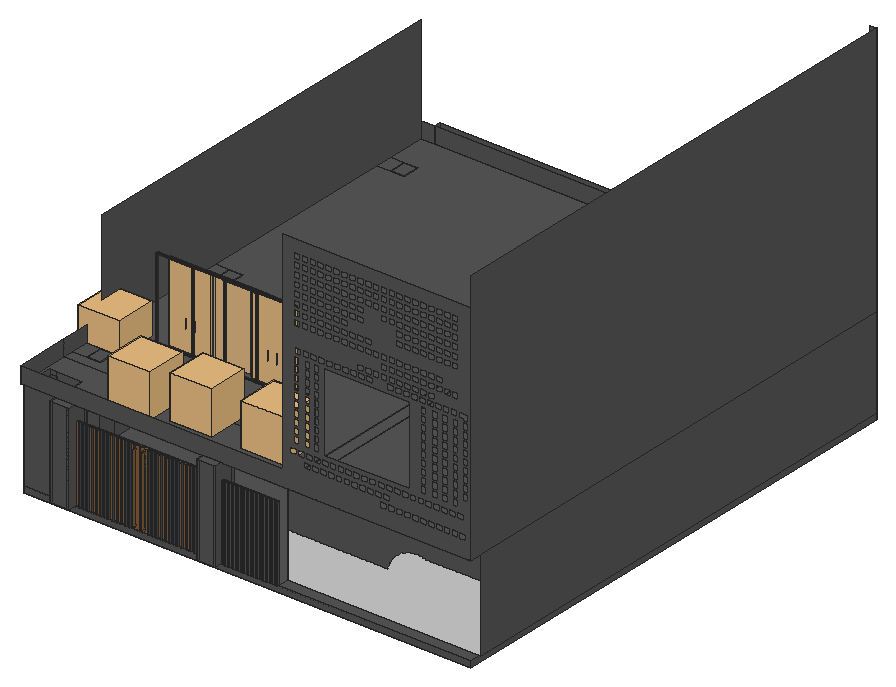
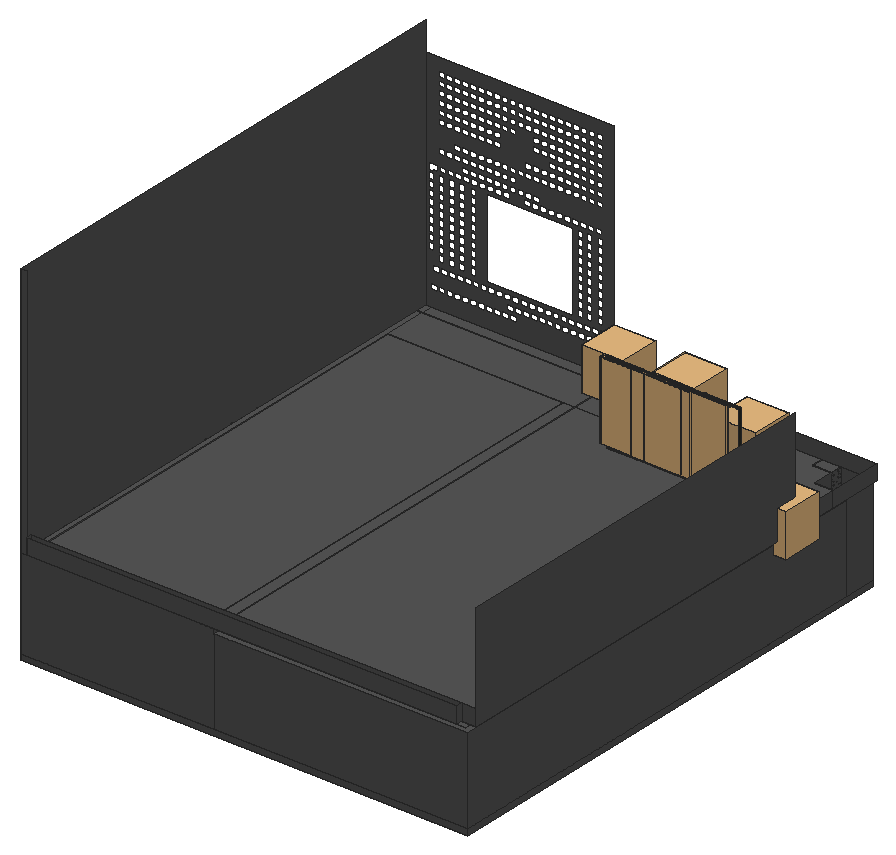
# SketchUp Ruby script. Lengths in inches.
U = 1.inch
M = Sketchup.active_model
def pt(a) = Geom::Point3d.new(a.map { |v| v * U })
def face(e, loops, mat)
  f = e.add_face(loops[0].map { |a| pt(a) })
  loops[1..].each { |l| e.add_face(l.map { |a| pt(a) }).erase! }
  f.material = f.back_material = mat if mat
  f
end
# faces: each face lists its corners as indices into pts; further lists are holes
def faces(e, pts, list, mat = nil) = list.each { |f| face(e, (f[0].is_a?(Array) ? f : [f]).map { |l| l.map { |i| pts[i] } }, mat) }
# xy, xz, yz: faces in a plane at the given z, y or x. An outline is a flat list of corners, or four numbers for a rectangle; further outlines are holes
def ring(l) = l.size == 4 ? [[l[0], l[1]], [l[2], l[1]], [l[2], l[3]], [l[0], l[3]]] : l.each_slice(2).to_a
def flat(e, list, mat, &to3) = list.each { |f| face(e, (f[0].is_a?(Array) ? f : [f]).map { |l| ring(l).map { |u, v| to3.(u, v) } }, mat) }
def xy(e, z, list, mat = nil) = flat(e, list, mat) { |x, y| [x, y, z] }
def xz(e, y, list, mat = nil) = flat(e, list, mat) { |x, z| [x, y, z] }
def yz(e, x, list, mat = nil) = flat(e, list, mat) { |y, z| [x, y, z] }
def lines(e, pts, list) = list.each { |a, b| e.add_line(pt(pts[a]), pt(pts[b])) }
# prism: a flat outline (further loops are holes) pulled along v
def prism(e, loops, v, mat = nil)
  f = face(e, loops, mat); d = Geom::Vector3d.new(v.map { |x| x * U })
  f.pushpull(f.normal.samedirection?(d) ? d.length : -d.length)
end
def box(e, o, s, mat = nil) = prism(e, [[o, [o[0] + s[0], o[1], o[2]], [o[0] + s[0], o[1] + s[1], o[2]], [o[0], o[1] + s[1], o[2]]]], [0, 0, s[2]], mat)
def at(x, y, z, deg = 0) = Geom::Transformation.translation(pt([x, y, z])) * Geom::Transformation.rotation(ORIGIN, Z_AXIS, deg.degrees)
def axes(o, x, y, z) = Geom::Transformation.new([*x, 0, *y, 0, *z, 0, *pt(o).to_a, 1])
def part(name) = M.definitions.add(name)
# library, detail: a bought-in or finely detailed component or shape, given as its bounding box
def library(name, o, s) = part(name).tap { |d| box(d.entities, o, s) }
def detail(e, o, s) = box(e.add_group.entities, o, s)
def put(e, d, t, mat = nil) = e.add_instance(d, t).tap { |i| i.material = mat if mat }
def group(e, t, mat = nil) = e.add_group.tap { |g| g.transformation = t; g.material = mat if mat }.entities
root = M.entities
M.materials.add("48,62,1").color = [75, 79, 82]
M.materials.add("Glazing").color = [128, 128, 128]
M.materials["Glazing"].alpha = 0.05
M.materials.add("Powdercoating").color = [41, 44, 40]
M.materials.add("[Color M06]").color = [86, 86, 86]
M.materials.add("[Polished Concrete Old]").color = [229, 229, 229]
M.materials.add("hpl-fundermax-sheets-500x500").color = [131, 93, 58]
c1 = part("FLUTED+WOOD")
g1 = group(c1.entities,at(0,-21.52,1.9375))
prism(g1,[[[0,45.2,-1.9375],[0.5,45.2,-1.9375],[1,45.2,-1.9375],[1,21.53,-1.9375],[0.5,21.52,-1.9375],[0,21.52,-1.9375],[0,22.6,-1.9375],[0.5,22.6,-1.9375],[0.5,23.14,-1.9375],[0,23.14,-1.9375],[0,24.22,-1.9375],[0.5,24.22,-1.9375],[0.5,24.75,-1.9375],[0,24.75,-1.9375],[0,25.83,-1.9375],[0.5,25.83,-1.9375],[0.5,26.37,-1.9375],[0,26.37,-1.9375],[0,27.44,-1.9375],[0.5,27.44,-1.9375],[0.5,27.98,-1.9375],[0,27.98,-1.9375],[0,29.06,-1.9375],[0.5,29.06,-1.9375],[0.5,29.6,-1.9375],[0,29.6,-1.9375],[0,30.67,-1.9375],[0.5,30.67,-1.9375],[0.5,31.21,-1.9375],[0,31.21,-1.9375],[0,32.29,-1.9375],[0.5,32.29,-1.9375],[0.5,32.83,-1.9375],[0,32.83,-1.9375],[0,33.9,-1.9375],[0.5,33.9,-1.9375],[0.5,34.44,-1.9375],[0,34.44,-1.9375],[0,35.52,-1.9375],[0.5,35.52,-1.9375],[0.5,36.05,-1.9375],[0,36.05,-1.9375],[0,37.13,-1.9375],[0.5,37.13,-1.9375],[0.5,37.67,-1.9375],[0,37.67,-1.9375],[0,38.75,-1.9375],[0.5,38.74,-1.9375],[0.5,39.28,-1.9375],[0,39.28,-1.9375],[0,40.36,-1.9375],[0.5,40.36,-1.9375],[0.5,40.9,-1.9375],[0,40.9,-1.9375],[0,41.97,-1.9375],[0.5,41.97,-1.9375],[0.5,42.51,-1.9375],[0,42.51,-1.9375],[0,43.59,-1.9375],[0.5,43.59,-1.9375],[0.5,44.125,-1.9375],[0,44.125,-1.9375]]],[0,0,46.125])
c2 = part("Group\#60")
prism(c2.entities,[[[-0.75,0,69],[-0.75,0,68],[-0.75,-1.375,68],[-0.75,-1.375,4],[-0.75,0,4],[-0.75,0,3],[-0.75,-2.75,3],[-0.75,-2.75,69]]],[1.5,0,0])
c3 = part("Group\#59")
box(c3.entities,[0,-0.75,0],[0.75,0.75,72])
c4 = part("Gate")
g2 = group(c4.entities,at(0,0,0))
g3 = group(g2,at(12,3,0))
prism(g3,[[[1.5,-3,0],[3,-3,0],[3,12,0],[-12,12,0],[-12,-3,0],[-10.5,-3,0]]],[0,0,72])
prism(g3,[[[118.5,-3,0],[120,-3,0],[120,12,0],[105,12,0],[105,-3,0],[106.5,-3,0]]],[0,0,72])
g4 = group(g2,at(121,6.75,0),"hpl-fundermax-sheets-500x500")
xy(g4,0,[[-106.75,0,-55.38,2],[-54.93,0,-4,2]])
xy(g4,60,[[-106.75,0,-55.38,2],[-54.93,0,-4,2]])
xz(g4,0,[[-106.75,0,-59.6,60],[-58.9375,0,-55.38,60],[-54.93,0,-51.375,60],[-50.71,0,-48.04,60],[-47.37,0,-4,60]])
xz(g4,0,[[-59.6,0,-58.9375,60],[-51.375,0,-50.71,60]],"48,62,1")
xz(g4,2,[[-106.75,0,-55.38,60],[-54.93,0,-4,60]])
yz(g4,-106.75,[[0,0,2,60]])
yz(g4,-55.38,[[0,0,2,60]])
yz(g4,-54.93,[[0,0,2,60]])
yz(g4,-4,[[0,0,2,60]])
put(g4,c2,axes([-51.6,0,0],[-0.88961,0,0],[0,1,0],[0,0,0.83333]))
put(g4,c2,axes([-58.71,0,0],[-0.88961,0,0],[0,1,0],[0,0,0.83333]))
put(g4,c3,axes([-47.37,0,0],[-0.88961,0,0],[0,1,0],[0,0,0.83333]),"48,62,1")
put(g4,c3,axes([-44.04,0,0],[-0.88961,0,0],[0,1,0],[0,0,0.83333]),"48,62,1")
put(g4,c3,axes([-40.7,0,0],[-0.88961,0,0],[0,1,0],[0,0,0.83333]),"48,62,1")
put(g4,c3,axes([-37.36,0,0],[-0.88961,0,0],[0,1,0],[0,0,0.83333]),"48,62,1")
put(g4,c3,axes([-34.03,0,0],[-0.88961,0,0],[0,1,0],[0,0,0.83333]),"48,62,1")
put(g4,c3,axes([-30.69,0,0],[-0.88961,0,0],[0,1,0],[0,0,0.83333]),"48,62,1")
put(g4,c3,axes([-27.36,0,0],[-0.88961,0,0],[0,1,0],[0,0,0.83333]),"48,62,1")
put(g4,c3,axes([-24.02,0,0],[-0.88961,0,0],[0,1,0],[0,0,0.83333]),"48,62,1")
put(g4,c3,axes([-20.68,0,0],[-0.88961,0,0],[0,1,0],[0,0,0.83333]),"48,62,1")
put(g4,c3,axes([-17.35,0,0],[-0.88961,0,0],[0,1,0],[0,0,0.83333]),"48,62,1")
put(g4,c3,axes([-14.01,0,0],[-0.88961,0,0],[0,1,0],[0,0,0.83333]),"48,62,1")
put(g4,c3,axes([-10.68,0,0],[-0.88961,0,0],[0,1,0],[0,0,0.83333]),"48,62,1")
put(g4,c3,axes([-7.34,0,0],[-0.88961,0,0],[0,1,0],[0,0,0.83333]),"48,62,1")
put(g4,c3,axes([-4,0,0],[-0.88961,0,0],[0,1,0],[0,0,0.83333]),"48,62,1")
put(g4,c3,axes([-62.27,0,0],[-0.88961,0,0],[0,1,0],[0,0,0.83333]),"48,62,1")
put(g4,c3,axes([-65.61,0,0],[-0.88961,0,0],[0,1,0],[0,0,0.83333]),"48,62,1")
put(g4,c3,axes([-68.94,0,0],[-0.88961,0,0],[0,1,0],[0,0,0.83333]),"48,62,1")
put(g4,c3,axes([-72.28,0,0],[-0.88961,0,0],[0,1,0],[0,0,0.83333]),"48,62,1")
put(g4,c3,axes([-75.62,0,0],[-0.88961,0,0],[0,1,0],[0,0,0.83333]),"48,62,1")
put(g4,c3,axes([-78.95,0,0],[-0.88961,0,0],[0,1,0],[0,0,0.83333]),"48,62,1")
put(g4,c3,axes([-82.29,0,0],[-0.88961,0,0],[0,1,0],[0,0,0.83333]),"48,62,1")
put(g4,c3,axes([-85.625,0,0],[-0.88961,0,0],[0,1,0],[0,0,0.83333]),"48,62,1")
put(g4,c3,axes([-88.96,0,0],[-0.88961,0,0],[0,1,0],[0,0,0.83333]),"48,62,1")
put(g4,c3,axes([-92.3,0,0],[-0.88961,0,0],[0,1,0],[0,0,0.83333]),"48,62,1")
put(g4,c3,axes([-95.63,0,0],[-0.88961,0,0],[0,1,0],[0,0,0.83333]),"48,62,1")
put(g4,c3,axes([-98.97,0,0],[-0.88961,0,0],[0,1,0],[0,0,0.83333]),"48,62,1")
put(g4,c3,axes([-102.31,0,0],[-0.88961,0,0],[0,1,0],[0,0,0.83333]),"48,62,1")
put(g4,c3,axes([-106.09,0,0],[-0.88961,0,0],[0,1,0],[0,0,0.83333]),"48,62,1")
c5 = library("Pot+Plant",[-20.81,-17.08,-0.03],[39.86,39.43,41.33])
c6 = part("Group\#15")
xy(c6.entities,0,[[0,-55.94,0.71,45.94]])
xy(c6.entities,0.2,[[0,-55.94,0.47,45.94],[0.47,45.94,0.71,46.42]])
xy(c6.entities,2.36,[[0.47,-55.94,0.71,46.42]])
xz(c6.entities,-55.94,[[0,0,0.71,0,0.71,2.36,0.47,2.36,0.47,0.2,0,0.2]])
xz(c6.entities,45.94,[[0,0,0.71,0.2]])
xz(c6.entities,46.42,[[0.47,0.2,0.71,2.36]])
yz(c6.entities,0,[[-55.94,0,45.94,0.2]])
yz(c6.entities,0.47,[[-55.94,0.2,46.42,2.36]])
yz(c6.entities,0.71,[[-55.94,0,45.94,0,45.94,0.2,46.42,0.2,46.42,2.36,-55.94,2.36]])
c7 = part("Group\#7")
xy(c7.entities,0,[[0,-59.09,0.71,45.94]])
xy(c7.entities,0.2,[[0,-59.09,0.47,45.94],[0.47,45.94,0.71,46.42]])
xy(c7.entities,2.36,[[0.47,-59.09,0.71,46.42]])
xz(c7.entities,-59.09,[[0,0,0.71,0,0.71,2.36,0.47,2.36,0.47,0.2,0,0.2]])
xz(c7.entities,45.94,[[0,0,0.71,0.2]])
xz(c7.entities,46.42,[[0.47,0.2,0.71,2.36]])
yz(c7.entities,0,[[-59.09,0,45.94,0.2]])
yz(c7.entities,0.47,[[-59.09,0.2,46.42,2.36]])
yz(c7.entities,0.71,[[-59.09,0,45.94,0,45.94,0.2,46.42,0.2,46.42,2.36,-59.09,2.36]])
c8 = part("Group\#16")
prism(c8.entities,[[[0.47,-56.18,0.2],[0,-56.18,0.2],[0,-56.18,0],[0.71,-56.18,0],[0.71,-56.18,2.36],[0.47,-56.18,2.36]]],[0,28.68,0])
c9 = part("Group\#10")
box(c9.entities,[-0.73,0,0],[27.99,0.55,102.05])
c10 = part("Group\#18")
xy(c10.entities,0,[[0.47,-56.18,0.47,-55.47,0,-55.47,0,-28.21,1.18,-28.21,1.18,-56.18]])
xy(c10.entities,0.2,[[0.71,-56.18,1.18,-28.21],[0,-55.47,0.47,-28.21],[0.47,-28.21,0.71,-27.74]])
xy(c10.entities,2.36,[[0.47,-56.18,0.71,-27.74]])
xz(c10.entities,-56.18,[[0.47,0,1.18,0,1.18,0.2,0.71,0.2,0.71,2.36,0.47,2.36]])
xz(c10.entities,-55.47,[[0,0,0.47,0.2]])
xz(c10.entities,-28.21,[[0,0,1.18,0.2]])
xz(c10.entities,-27.74,[[0.47,0.2,0.71,2.36]])
yz(c10.entities,0,[[-55.47,0,-28.21,0.2]])
yz(c10.entities,0.47,[[-56.18,0,-55.47,0.2],[-56.18,0.2,-27.74,2.36]])
yz(c10.entities,0.71,[[-56.18,0.2,-27.74,2.36]])
yz(c10.entities,1.18,[[-56.18,0,-28.21,0.2]])
c11 = part("Group\#34")
xy(c11.entities,0,[[-20.45,0,7.76,1.22]])
xy(c11.entities,0.06,[[-20.39,0.06,7.7,1.22]])
xy(c11.entities,0.47,[[-19.98,0,7.28,0.06]])
xy(c11.entities,101.89,[[-19.98,0,7.28,0.06]])
xy(c11.entities,102.3,[[-20.39,0.06,7.7,1.22]])
xy(c11.entities,102.36,[[-20.45,0,7.76,1.22]])
xz(c11.entities,0,[[[-20.45,0,7.76,102.36],[-19.98,0.47,7.28,101.89]]])
xz(c11.entities,0.06,[[[-20.39,0.06,7.7,102.3],[-19.98,0.47,7.28,101.89]]])
xz(c11.entities,1.22,[[[-20.45,0,7.76,102.36],[-20.39,0.06,7.7,102.3]]])
yz(c11.entities,-20.45,[[0,0,1.22,102.36]])
yz(c11.entities,-20.39,[[0.06,0.06,1.22,102.3]])
yz(c11.entities,-19.98,[[0,0.47,0.06,101.89]])
yz(c11.entities,7.28,[[0,0.47,0.06,101.89]])
yz(c11.entities,7.7,[[0.06,0.06,1.22,102.3]])
yz(c11.entities,7.76,[[0,0,1.22,102.36]])
c12 = part("Group\#6")
put(c12.entities,c6,axes([27.97,0,7.875],[1,0,0],[0,0,-1],[0,1,0]),"Powdercoating")
put(c12.entities,c7,axes([0.71,0,6.8],[-1,0,0],[0,0,-0.97687],[0,1,0]),"Powdercoating")
put(c12.entities,c8,axes([-27.5,0,-38.07],[0,0,-1],[-1,0,0],[0,1,0]),"Powdercoating")
put(c12.entities,c9,at(1.12,0.35,-38.39),"Glazing")
put(c12.entities,c10,axes([-27.5,0,63.35],[0,0,1],[-1,0,0],[0,1,0]),"Powdercoating")
put(c12.entities,c11,at(20.6875,1.0625,-38.54),"Powdercoating")
c13 = part("Sliding door panels")
put(c13.entities,c12,at(-1.18,4.5,38.86))
g5 = group(c13.entities,at(84.74,4.5,38.86))
put(g5,c6,axes([-27.97,0,7.875],[-1,0,0],[0,0,-1],[0,1,0]),"Powdercoating")
put(g5,c7,axes([-0.71,0,6.8],[1,0,0],[0,0,-0.97687],[0,1,0]),"Powdercoating")
put(g5,c8,axes([27.5,0,-38.07],[0,0,-1],[1,0,0],[0,1,0]),"Powdercoating")
put(g5,c9,axes([-1.12,0.35,-38.39],[-1,0,0],[0,1,0],[0,0,1]),"Glazing")
put(g5,c10,axes([27.5,0,63.35],[0,0,1],[1,0,0],[0,1,0]),"Powdercoating")
put(g5,c11,axes([-20.6875,1.0625,-38.54],[-1,0,0],[0,1,0],[0,0,1]),"Powdercoating")
g6 = group(c13.entities,at(56.0625,4.5,38.86))
put(g6,c6,axes([-27.97,0,7.875],[-1,0,0],[0,0,-1],[0,1,0]),"Powdercoating")
put(g6,c8,axes([27.5,0,-38.07],[0,0,-1],[1,0,0],[0,1,0]),"Powdercoating")
put(g6,c9,axes([-1.12,0.35,-38.39],[-1,0,0],[0,1,0],[0,0,1]),"Glazing")
put(g6,c10,axes([27.5,0,63.35],[0,0,1],[1,0,0],[0,1,0]),"Powdercoating")
put(g6,c11,axes([-20.6875,1.0625,-38.54],[-1,0,0],[0,1,0],[0,0,1]),"Powdercoating")
g7 = group(g6,at(-0.71,0,6.8),"Powdercoating")
xy(g7,-45.34,[[0.47,0.2,0.71,2.36]])
xy(g7,-44.88,[[0,0,0.71,0.2]])
xy(g7,57.73,[[0,0,0.71,0,0.71,2.36,0.47,2.36,0.47,0.2,0,0.2]])
xz(g7,0,[[0,-44.88,0.71,57.73]])
xz(g7,0.2,[[0.47,-45.34,0.71,-44.88],[0,-44.88,0.47,57.73]])
xz(g7,2.36,[[0.47,-45.34,0.71,57.73]])
yz(g7,0,[[0,-44.88,0.2,57.73]])
yz(g7,0.47,[[0.2,-45.34,2.36,57.73]])
yz(g7,0.71,[[0.2,-45.34,2.36,-45.34,2.36,57.73,0,57.73,0,-44.88,0.2,-44.88]])
put(c13.entities,c12,axes([-33.94,4.5,38.86],[1.14218,0,0],[0,1,0],[0,0,1]))
c14 = part("sliding door")
put(c14.entities,c13,at(0,-4.5,-0.08))
c15 = library("Group14",[-64.97,9.24,0.31],[138.52,9.93,292.57])
c16 = library("Group16",[86.37,-10.76,76.46],[21.79,14.87,35.97])
c17 = library("Group22",[48.82,-10.91,0.23],[97.72,18.57,293.12])
c18 = library("Group24",[44.03,2.01,0.26],[103.73,11,292.35])
c19 = library("Group27",[-106.21,-10.76,76.46],[21.8,14.87,35.97])
c20 = library("Group35",[-145.81,2.01,0.26],[103.73,11,292.35])
c21 = library("Group33",[-144.59,-10.91,0.23],[97.72,18.57,293.12])
c22 = part("rem")
g8 = group(c22.entities,at(-145.81,-10.91,0.23))
put(g8,c15,at(145.81,10.91,-0.23))
put(g8,c16,at(145.81,10.91,-0.23))
put(g8,c17,at(145.81,10.91,-0.23))
put(g8,c18,at(145.81,10.91,-0.23))
put(g8,c19,at(145.81,10.91,-0.23))
put(g8,c20,at(145.81,10.91,-0.23))
put(g8,c21,at(145.81,10.91,-0.23))
xy(root,108.9,[[5.91,10.05,600.47,683.05]],"[Color M06]")
xy(root,116.71,[[5.91,10.05,48.91,53.05],[[48.91,10.05,48.91,53.05,15.35,53.05,15.35,675.01,343.85,675.01,343.85,10.05,266.81,10.05,266.81,32.55,248.56,32.55,248.56,10.05],[19.84,601.77,37.72,624.46],[19.84,311.33,37.72,334.02],[19.84,97.21,37.72,119.89]],[248.56,10.05,266.81,32.55],[343.85,10.05,600.47,25.42],[[343.85,25.42,600.47,683.05],[359.6,82.9,592.4375,675.01]],
  [5.91,53.05,15.35,675.01],[359.6,82.9,592.4375,675.01],[5.91,675.01,343.85,683.05]],"[Color M06]")
xy(root,230.71,[[5.91,53.05,15.35,53.05,15.35,675.01,343.85,675.01,343.85,683.05,5.91,683.05]],"[Color M06]")
xy(root,236.71,[[1.28,10.05,1.28,82.9,343.85,82.9,343.85,10.05,266.81,10.05,266.81,32.55,248.56,32.55,248.56,10.05,48.91,10.05,48.91,53.05,5.91,53.05,5.91,10.05],[343.85,10.05,592.4375,25.42],[592.4375,10.05,600.47,25.42],[343.85,25.42,592.4375,82.9],[592.4375,25.42,600.47,683.05],
  [1.28,82.9,1.28,97.21,37.72,97.21,37.72,119.89,1.28,119.89,1.28,311.33,37.72,311.33,37.72,334.02,1.28,334.02,1.28,601.77,37.72,601.77,37.72,624.46,1.28,624.46,1.28,675.01,343.85,675.01,343.85,82.9],[343.85,82.9,359.6,675.01],[359.6,82.9,592.4375,675.01],[1.28,97.21,19.84,119.89],[19.84,97.21,37.72,119.89],
  [1.28,311.33,19.84,334.02],[19.84,311.33,37.72,334.02],[1.28,601.77,19.84,624.46],[19.84,601.77,37.72,624.46],[19.84,675.01,343.85,683.05],
  [343.85,675.01,592.4375,683.05]],"[Color M06]")
xz(root,10.05,[[5.91,108.9,600.47,116.71],[5.91,116.71,48.91,236.71],[248.56,116.71,266.81,236.71],[[1.28,236.71,600.47,236.71,600.47,537.58,349.9,537.58,349.9,257.83,1.28,257.83],[404.15,292.65,518.59,397.33],[589.18,398.91,589.18,401.04,583.39,401.04,583.39,408.36,592.39,408.36,592.39,407.91,596.49,407.91,596.49,398.91],[364.36,513.93,373.36,521.25],[374.86,513.93,383.86,521.25],[385.36,513.93,394.36,521.25],[395.86,513.93,404.86,521.25],[406.36,513.93,415.36,521.25],[416.86,513.93,425.86,521.25],[427.36,513.93,436.36,521.25],[437.86,513.93,446.86,521.25],[448.36,513.93,457.36,521.25],[458.86,513.93,467.86,521.25],[469.36,513.93,478.36,521.25],[479.86,513.93,488.86,521.25],[490.36,513.93,499.36,521.25],[500.86,513.93,509.86,521.25],[511.36,513.93,520.36,521.25],[521.86,513.93,530.86,521.25],[532.36,513.93,541.36,521.25],[542.86,513.93,551.86,521.25],[553.36,513.93,562.36,521.25],[563.86,513.93,572.86,521.25],[574.36,513.93,583.36,521.25],[574.36,503,583.36,510.31],[563.86,503,572.86,510.31],[553.36,503,562.36,510.31],[542.86,503,551.86,510.31],[532.36,503,541.36,510.31],[521.86,503,530.86,510.31],[511.36,503,520.36,510.31],[500.86,503,509.86,510.31],[490.36,503,499.36,510.31],[479.86,503,488.86,510.31],[469.36,503,478.36,510.31],[458.86,503,467.86,510.31],[448.36,503,457.36,510.31],[437.86,503,446.86,510.31],[427.36,503,436.36,510.31],[416.86,503,425.86,510.31],[406.36,503,415.36,510.31],[395.86,503,404.86,510.31],[385.36,503,394.36,510.31],[374.86,503,383.86,510.31],[364.36,503,373.36,510.31],[574.36,491.43,583.36,498.75],[563.86,491.43,572.86,498.75],[553.36,491.43,562.36,498.75],[542.86,491.43,551.86,498.75],[532.36,491.43,541.36,498.75],[521.86,491.43,530.86,498.75],[511.36,491.43,520.36,498.75],[500.86,491.43,509.86,498.75],[490.36,491.43,499.36,498.75],[479.86,491.43,488.86,498.75],[469.36,491.43,478.36,498.75],[458.86,491.43,467.86,498.75],[448.36,491.43,457.36,498.75],[437.86,491.43,446.86,498.75],[427.36,491.43,436.36,498.75],[416.86,491.43,425.86,498.75],[406.36,491.43,415.36,498.75],[395.86,491.43,404.86,498.75],[385.36,491.43,394.36,498.75],[374.86,491.43,383.86,498.75],[364.36,491.43,373.36,498.75],[574.36,479.87,583.36,487.18],[563.86,479.87,572.86,487.18],[553.36,479.87,562.36,487.18],[542.86,479.87,551.86,487.18],[532.36,479.87,541.36,487.18],[521.86,479.87,530.86,487.18],[511.36,479.87,520.36,487.18],[500.86,479.87,509.86,487.18],[448.36,479.87,457.36,487.18],[437.86,479.87,446.86,487.18],[427.36,479.87,436.36,487.18],[416.86,479.87,425.86,487.18],[406.36,479.87,415.36,487.18],[395.86,479.87,404.86,487.18],[385.36,479.87,394.36,487.18],[374.86,479.87,383.86,487.18],[364.36,479.87,373.36,487.18],[574.36,468.43,583.36,475.75],[563.86,468.43,572.86,475.75],[553.36,468.43,562.36,475.75],[542.86,468.43,551.86,475.75],[532.36,468.43,541.36,475.75],[521.86,468.43,530.86,475.75],[511.36,468.43,520.36,475.75],[500.86,468.43,509.86,475.75],[448.36,468.43,457.36,475.75],[437.86,468.43,446.86,475.75],[427.36,468.43,436.36,475.75],[416.86,468.43,425.86,475.75],[406.36,468.43,415.36,475.75],[395.86,468.43,404.86,475.75],[385.36,468.43,394.36,475.75],[374.86,468.43,383.86,475.75],[364.36,468.43,373.36,475.75],[574.36,457,583.36,464.31],[563.86,457,572.86,464.31],[553.36,457,562.36,464.31],[542.86,457,551.86,464.31],[532.36,457,541.36,464.31],[521.86,457,530.86,464.31],[511.36,457,520.36,464.31],[500.86,457,509.86,464.31],[490.36,480,499.36,487.31],[479.86,480,488.86,487.31],[427.36,457,436.36,464.31],[416.86,457,425.86,464.31],[406.36,457,415.36,464.31],[395.86,457,404.86,464.31],[385.36,457,394.36,464.31],[374.86,457,383.86,464.31],[364.36,457,373.36,464.31],[458.86,445.43,467.86,452.75],[448.36,445.43,457.36,452.75],[437.86,445.43,446.86,452.75],[427.36,445.43,436.36,452.75],[416.86,445.43,425.86,452.75],[406.36,445.43,415.36,452.75],[395.86,445.43,404.86,452.75],[385.36,445.43,394.36,452.75],[374.86,445.43,383.86,452.75],[364.36,445.43,373.36,452.75],[553.36,433.87,562.36,441.18],[542.86,433.87,551.86,441.18],[532.36,433.87,541.36,441.18],[521.86,433.87,530.86,441.18],[511.36,433.87,520.36,441.18],[500.86,433.87,509.86,441.18],[490.36,433.87,499.36,441.18],[479.86,433.87,488.86,441.18],[469.36,433.87,478.36,441.18],[458.86,433.87,467.86,441.18],[448.36,433.87,457.36,441.18],[437.86,433.87,446.86,441.18],[427.36,433.87,436.36,441.18],[416.86,433.87,425.86,441.18],[406.36,433.87,415.36,441.18],[395.86,433.87,404.86,441.18],[385.36,433.87,394.36,441.18],[374.86,433.87,383.86,441.18],[364.36,433.87,373.36,441.18],[574.36,422.31,583.36,429.62],[563.86,422.31,572.86,429.62],[553.36,422.31,562.36,429.62],[542.86,422.31,551.86,429.62],[532.36,422.31,541.36,429.62],[521.86,422.31,530.86,429.62],[511.36,422.31,520.36,429.62],[500.86,422.31,509.86,429.62],[490.36,422.31,499.36,429.62],[479.86,422.31,488.86,429.62],[542.86,410.43,551.86,417.74],[532.36,410.43,541.36,417.74],[521.86,410.43,530.86,417.74],[511.36,410.43,520.36,417.74],[500.86,410.43,509.86,417.74],[490.36,410.43,499.36,417.74],[479.86,410.43,488.86,417.74],[469.36,410.43,478.36,417.74],[458.86,410.43,467.86,417.74],[448.36,410.43,457.36,417.74],[460.14,401.04,469.14,408.36],[449.64,401.04,458.64,408.36],[439.14,401.04,448.14,408.36],[428.64,401.04,437.64,408.36],[418.14,401.04,427.14,408.36],[407.64,401.04,416.64,408.36],[397.14,401.04,406.14,408.36],[386.64,401.04,395.64,408.36],[376.14,401.04,385.14,408.36],[365.64,401.04,374.64,408.36],[572.89,401.04,581.89,408.36],[562.39,401.04,571.39,408.36],[551.89,401.04,560.89,408.36],[541.39,401.04,550.39,408.36],[530.89,401.04,539.89,408.36],[520.39,401.04,529.39,408.36],[509.89,401.04,518.89,408.36],[499.39,401.04,508.39,408.36],[488.89,401.04,497.89,408.36],[589.18,304.41,596.49,313.41],[589.18,314.91,596.49,323.91],[589.18,325.41,596.49,334.41],[589.18,335.91,596.49,344.91],[589.18,346.41,596.49,355.41],[589.18,356.91,596.49,365.91],[589.18,367.41,596.49,376.41],[589.18,377.91,596.49,386.91],[589.18,388.41,596.49,397.41],[575.62,388.24,582.93,397.24],[575.62,335.74,582.93,344.74],[575.62,367.24,582.93,376.24],[575.62,293.74,582.93,302.74],[575.62,346.24,582.93,355.24],[575.62,314.74,582.93,323.74],[575.62,377.74,582.93,386.74],[575.62,325.24,582.93,334.24],[575.62,356.74,582.93,365.74],[575.62,304.24,582.93,313.24],[561.81,388.24,569.12,397.24],[561.81,346.24,569.12,355.24],[561.81,293.74,569.12,302.74],[561.81,377.74,569.12,386.74],[561.81,367.24,569.12,376.24],[561.81,335.74,569.12,344.74],[561.81,325.24,569.12,334.24],[561.81,356.74,569.12,365.74],[561.81,314.74,569.12,323.74],[561.81,304.24,569.12,313.24],[548.43,388.24,555.74,397.24],[548.43,377.74,555.74,386.74],[548.43,304.24,555.74,313.24],[548.43,367.24,555.74,376.24],[548.43,356.74,555.74,365.74],[548.43,293.74,555.74,302.74],[548.43,335.74,555.74,344.74],[548.43,325.24,555.74,334.24],[548.43,314.74,555.74,323.74],[548.43,346.24,555.74,355.24],[532.99,388.24,540.31,397.24],[532.99,293.74,540.31,302.74],[532.99,335.74,540.31,344.74],[532.99,325.24,540.31,334.24],[532.99,314.74,540.31,323.74],[532.99,377.74,540.31,386.74],[532.99,304.24,540.31,313.24],[532.99,356.74,540.31,365.74],[532.99,346.24,540.31,355.24],[532.99,367.24,540.31,376.24],[390.99,388.24,398.31,397.24],[390.99,293.74,398.31,302.74],[390.99,335.74,398.31,344.74],[390.99,314.74,398.31,323.74],[390.99,377.74,398.31,386.74],[390.99,325.24,398.31,334.24],[390.99,304.24,398.31,313.24],[390.99,367.24,398.31,376.24],[390.99,356.74,398.31,365.74],[390.99,346.24,398.31,355.24],[378.93,388.24,386.24,397.24],[378.93,293.74,386.24,302.74],[378.93,335.74,386.24,344.74],[378.93,314.74,386.24,323.74],[378.93,377.74,386.24,386.74],[378.93,325.24,386.24,334.24],[378.93,356.74,386.24,365.74],[378.93,367.24,386.24,376.24],[378.93,304.24,386.24,313.24],[378.93,346.24,386.24,355.24],[364.31,388.24,371.62,397.24],[364.31,367.24,371.62,376.24],[364.31,304.24,371.62,313.24],[364.31,346.24,371.62,355.24],[364.31,356.74,371.62,365.74],[364.31,293.74,371.62,302.74],[364.31,377.74,371.62,386.74],[364.31,335.74,371.62,344.74],[364.31,325.24,371.62,334.24],[364.31,314.74,371.62,323.74],[464.62,280.4375,473.62,287.75],[454.12,280.4375,463.12,287.75],[443.62,280.4375,452.62,287.75],[433.12,280.4375,442.12,287.75],[422.62,280.4375,431.62,287.75],[412.12,280.4375,421.12,287.75],[401.62,280.4375,410.62,287.75],[391.12,280.4375,400.12,287.75],[380.62,280.4375,389.62,287.75],[370.12,280.4375,379.12,287.75],[359.62,280.4375,368.62,287.75],[581.43,280.4375,590.43,287.75],[570.93,280.4375,579.93,287.75],[560.43,280.4375,569.43,287.75],[549.93,280.4375,558.93,287.75],[539.43,280.4375,548.43,287.75],[528.93,280.4375,537.93,287.75],[518.43,280.4375,527.43,287.75],[507.93,280.4375,516.93,287.75],[497.43,280.4375,506.43,287.75],[486.93,280.4375,495.93,287.75],[476.43,280.4375,485.43,287.75],[483.09,268.5,492.09,275.81],[472.59,268.5,481.59,275.81],[462.09,268.5,471.09,275.81],[451.59,268.5,460.59,275.81],[441.09,268.5,450.09,275.81],[430.59,268.5,439.59,275.81],[420.09,268.5,429.09,275.81],[409.59,268.5,418.59,275.81],[399.09,268.5,408.09,275.81],[388.59,268.5,397.59,275.81],[378.09,268.5,387.09,275.81],[584.61,257.42,593.61,264.73],[574.11,257.42,583.11,264.73],[563.61,257.42,572.61,264.73],[553.11,257.42,562.11,264.73],[542.61,257.42,551.61,264.73],[532.11,257.42,541.11,264.73],[521.61,257.42,530.61,264.73],[511.11,257.42,520.11,264.73],[500.61,257.42,509.61,264.73],[490.11,257.42,499.11,264.73],[479.61,257.42,488.61,264.73]]],"[Color M06]")
xz(root,25.42,[[343.85,176.71,477.48,176.71,479.14,181.88,481.47,186.79,484.45,191.33,488.01,195.43,492.09,199.01,496.62,202.01,501.51,204.375,506.67,206.05,512.02,207.02,517.44,207.26,522.85,206.76,528.15,205.54,600.47,205.54,600.47,236.71,343.85,236.71]],"[Color M06]")
xz(root,25.42,[[343.85,116.71,600.47,116.71,600.47,205.54,528.15,205.54,522.85,206.76,517.44,207.26,512.02,207.02,506.67,206.05,501.51,204.375,496.62,202.01,492.09,199.01,488.01,195.43,484.45,191.33,481.47,186.79,479.14,181.88,477.48,176.71,343.85,176.71]],"[Polished Concrete Old]")
xz(root,32.55,[[248.56,116.71,266.81,236.71]],"[Color M06]")
xz(root,53.05,[[5.91,116.71,15.35,230.71],[15.35,116.71,48.91,236.71],[5.91,230.71,15.35,236.71]],"[Color M06]")
xz(root,82.9,[[359.6,116.71,592.4375,236.71]],"[Color M06]")
xz(root,97.21,[[19.84,116.71,37.72,236.71]],"[Color M06]")
xz(root,119.89,[[19.84,116.71,37.72,236.71]],"[Color M06]")
xz(root,311.33,[[19.84,116.71,37.72,236.71]],"[Color M06]")
xz(root,334.02,[[19.84,116.71,37.72,236.71]],"[Color M06]")
xz(root,601.77,[[19.84,116.71,37.72,236.71]],"[Color M06]")
xz(root,624.46,[[19.84,116.71,37.72,236.71]],"[Color M06]")
xz(root,675.01,[[15.35,116.71,343.85,230.71],[359.6,116.71,592.4375,236.71],[1.28,236.71,19.84,257.83],[19.84,236.71,592.4375,257.83]],"[Color M06]")
xz(root,683.05,[[5.91,108.9,600.47,116.71],[5.91,116.71,343.85,230.71],[343.85,116.71,600.47,236.71],[19.84,236.71,592.4375,257.83],[592.4375,236.71,600.47,575.27]],"[Color M06]")
yz(root,1.28,[[10.05,236.71,82.9,257.83],[82.9,236.71,82.9,257.83,145.99,257.83,145.99,377.83,675.01,377.83,675.01,236.71]],"[Color M06]")
yz(root,5.91,[[10.05,108.9,683.05,116.71],[10.05,116.71,53.05,236.71],[53.05,116.71,683.05,230.71]],"[Color M06]")
yz(root,15.35,[[53.05,116.71,675.01,230.71]],"[Color M06]")
yz(root,19.84,[[97.21,116.71,119.89,236.71],[311.33,116.71,334.02,236.71],[601.77,116.71,624.46,236.71],[675.01,236.71,683.05,257.83]],"[Color M06]")
yz(root,37.72,[[97.21,116.71,119.89,236.71],[311.33,116.71,334.02,236.71],[601.77,116.71,624.46,236.71]],"[Color M06]")
yz(root,48.91,[[10.05,116.71,53.05,236.71]],"[Color M06]")
yz(root,248.56,[[10.05,116.71,32.55,236.71]],"[Color M06]")
yz(root,266.81,[[10.05,116.71,32.55,236.71]],"[Color M06]")
yz(root,343.85,[[25.42,116.71,82.9,236.71],[82.9,116.71,675.01,236.71],[675.01,230.71,683.05,236.71]],"[Color M06]")
yz(root,359.6,[[82.9,116.71,675.01,236.71]],"[Color M06]")
yz(root,592.4375,[[82.9,116.71,675.01,236.71],[675.01,236.71,683.05,257.83]],"[Color M06]")
yz(root,600.47,[[10.05,108.9,683.05,116.71],[25.42,116.71,683.05,236.71],[10.05,236.71,683.05,575.27]],"[Color M06]")
put(root,c1,axes([343.45,8.88,116.71],[0,2.17,0],[-3.1248,0,0],[0,0,2.17]),"[Color M06]")
put(root,c4,axes([48.91,0,116.71],[1.67,0,0],[0,1.67,0],[0,0,1.67]),"[Color M06]")
put(root,c5,axes([17.98,144.64,220.67],[1.38,0,0],[0,1.38,0],[0,0,1.38]))
put(root,c5,axes([128.47,56.67,237.07],[1.38,0,0],[0,1.38,0],[0,0,1.38]))
put(root,c14,axes([123.6,145.64,250.22],[1.47956,0,0],[0,1,0],[0,0,1.05053]),"[Color M06]")
put(root,c5,axes([312.875,46.57,253.45],[1.38,0,0],[0,1.38,0],[0,0,1.38]))
put(root,c5,axes([218.75,46.57,253.45],[1.38,0,0],[0,1.38,0],[0,0,1.38]))
put(root,c22,axes([172.23,148.07,254.05],[0.568,0,0],[0,0.19,0],[0,0,0.35379]),"[Color M06]")
